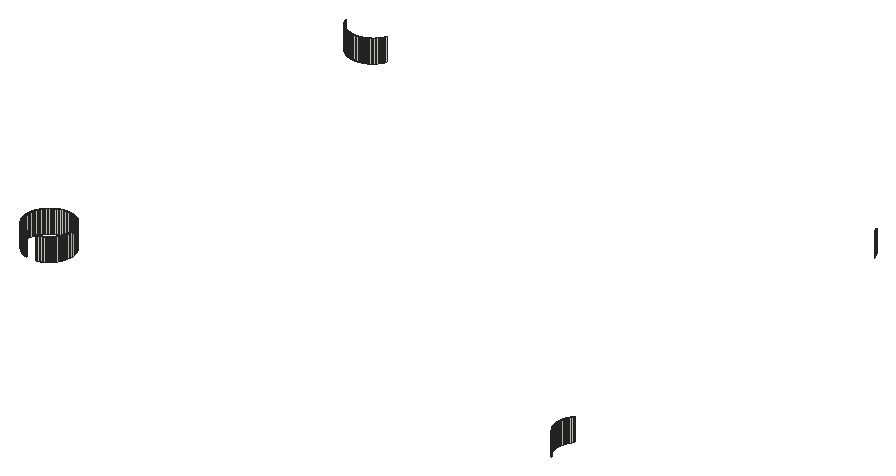
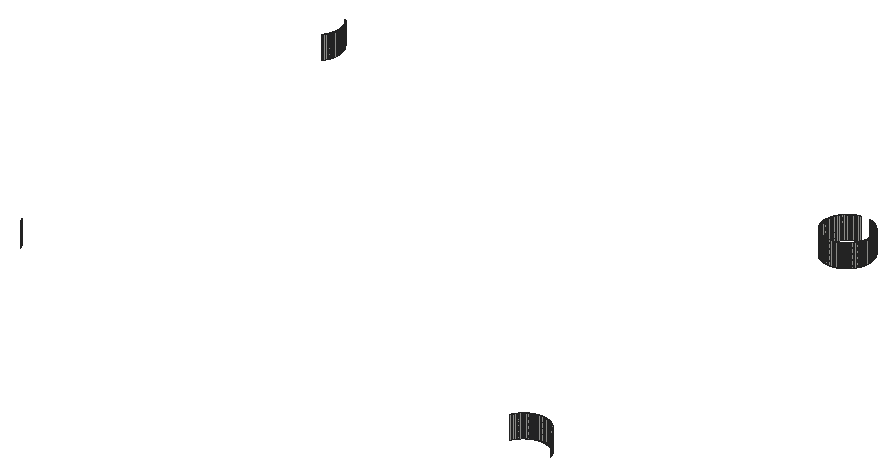
# SketchUp Ruby script. Lengths in inches.
U = 1.inch
M = Sketchup.active_model
def pt(a) = Geom::Point3d.new(a.map { |v| v * U })
def face(e, loops, mat)
  f = e.add_face(loops[0].map { |a| pt(a) })
  loops[1..].each { |l| e.add_face(l.map { |a| pt(a) }).erase! }
  f.material = f.back_material = mat if mat
  f
end
# faces: each face lists its corners as indices into pts; further lists are holes
def faces(e, pts, list, mat = nil) = list.each { |f| face(e, (f[0].is_a?(Array) ? f : [f]).map { |l| l.map { |i| pts[i] } }, mat) }
# xy, xz, yz: faces in a plane at the given z, y or x. An outline is a flat list of corners, or four numbers for a rectangle; further outlines are holes
def ring(l) = l.size == 4 ? [[l[0], l[1]], [l[2], l[1]], [l[2], l[3]], [l[0], l[3]]] : l.each_slice(2).to_a
def flat(e, list, mat, &to3) = list.each { |f| face(e, (f[0].is_a?(Array) ? f : [f]).map { |l| ring(l).map { |u, v| to3.(u, v) } }, mat) }
def xy(e, z, list, mat = nil) = flat(e, list, mat) { |x, y| [x, y, z] }
def xz(e, y, list, mat = nil) = flat(e, list, mat) { |x, z| [x, y, z] }
def yz(e, x, list, mat = nil) = flat(e, list, mat) { |y, z| [x, y, z] }
def lines(e, pts, list) = list.each { |a, b| e.add_line(pt(pts[a]), pt(pts[b])) }
# prism: a flat outline (further loops are holes) pulled along v
def prism(e, loops, v, mat = nil)
  f = face(e, loops, mat); d = Geom::Vector3d.new(v.map { |x| x * U })
  f.pushpull(f.normal.samedirection?(d) ? d.length : -d.length)
end
def box(e, o, s, mat = nil) = prism(e, [[o, [o[0] + s[0], o[1], o[2]], [o[0] + s[0], o[1] + s[1], o[2]], [o[0], o[1] + s[1], o[2]]]], [0, 0, s[2]], mat)
def at(x, y, z, deg = 0) = Geom::Transformation.translation(pt([x, y, z])) * Geom::Transformation.rotation(ORIGIN, Z_AXIS, deg.degrees)
def axes(o, x, y, z) = Geom::Transformation.new([*x, 0, *y, 0, *z, 0, *pt(o).to_a, 1])
def part(name) = M.definitions.add(name)
# library, detail: a bought-in or finely detailed component or shape, given as its bounding box
def library(name, o, s) = part(name).tap { |d| box(d.entities, o, s) }
def detail(e, o, s) = box(e.add_group.entities, o, s)
def put(e, d, t, mat = nil) = e.add_instance(d, t).tap { |i| i.material = mat if mat }
def group(e, t, mat = nil) = e.add_group.tap { |g| g.transformation = t; g.material = mat if mat }.entities
root = M.entities
xz(root,125,[[30.34,129,30.42,132],[30.42,129,30.5,132],[30.5,129,30.58,132],[30.58,129,30.66,132]])
xz(root,172.75,[[30.34,129,30.42,132],[30.42,129,30.5,132],[30.5,129,30.58,132],[30.58,129,30.66,132]])
yz(root,27.5,[[121.84,129,121.92,132],[121.92,129,122,132],[122,129,122.08,132],[122.08,129,122.16,132]])
yz(root,33.5,[[121.84,129,121.92,132],[121.92,129,122,132],[122,129,122.08,132],[122.08,129,122.16,132]])
yz(root,98,[[121.84,129,121.92,132],[121.92,129,122,132],[122,129,122.08,132],[122.08,129,122.16,132]])
p = [[29.57,119.15,129],[29.5,119.17,129],[29.5,119.17,132],[29.57,119.15,132],[29.72,119.1,129],[29.65,119.125,129],
  [29.65,119.125,132],[29.72,119.1,132],[29.8,119.08,129],[29.8,119.08,132],[29.875,119.07,129],[29.875,119.07,132],
  [31.125,119.07,129],[31.05,119.05,129],[31.05,119.05,132],[31.125,119.07,132],[31.2,119.08,129],[31.2,119.08,132],
  [31.28,119.1,129],[31.28,119.1,132],[31.35,119.125,129],[31.35,119.125,132],[31.43,119.15,129],[31.43,119.15,132],
  [31.5,119.17,129],[31.5,119.17,132],[29.35,119.23,129],[29.28,119.26,129],[29.28,119.26,132],[29.35,119.23,132],
  [29.42,119.2,129],[29.42,119.2,132],[31.58,119.2,129],[31.58,119.2,132],[31.65,119.23,129],[31.65,119.23,132],
  [31.72,119.26,129],[31.72,119.26,132],[29.21,119.29,129],[29.14,119.33,129],[29.14,119.33,132],[29.21,119.29,132],
  [29.07,119.36,129],[29.07,119.36,132],[31.79,119.29,129],[31.79,119.29,132],[31.86,119.33,129],[31.86,119.33,132],
  [31.93,119.36,129],[31.93,119.36,132],[29,119.4,129],[28.93,119.44,129],[28.93,119.44,132],[29,119.4,132],
  [28.87,119.48,129],[28.87,119.48,132],[32,119.4,129],[32,119.4,132],[32.07,119.44,129],[32.07,119.44,132],
  [32.13,119.48,129],[32.13,119.48,132],[28.8,119.53,129],[28.74,119.57,129],[28.74,119.57,132],[28.8,119.53,132],
  [32.2,119.53,129],[32.2,119.53,132],[32.26,119.57,129],[32.26,119.57,132],[28.67,119.62,129],[28.61,119.67,129],
  [28.61,119.67,132],[28.67,119.62,132],[32.33,119.62,129],[32.33,119.62,132],[32.39,119.67,129],[32.39,119.67,132],
  [28.55,119.72,129],[28.49,119.77,129],[28.49,119.77,132],[28.55,119.72,132],[32.45,119.72,129],[32.45,119.72,132],
  [32.51,119.77,129],[32.51,119.77,132],[28.43,119.82,129],[28.43,119.82,132],[28.38,119.88,129],[28.38,119.88,132],
  [32.57,119.82,129],[32.57,119.82,132],[32.62,119.88,129],[32.62,119.88,132],[28.32,119.93,129],[28.32,119.93,132],
  [28.27,119.99,129],[28.27,119.99,132],[32.68,119.93,129],[32.68,119.93,132],[32.73,119.99,129],[32.73,119.99,132],
  [28.22,120.05,129],[28.22,120.05,132],[32.78,120.05,129],[32.78,120.05,132],[28.17,120.11,129],[28.12,120.17,129],
  [28.12,120.17,132],[28.17,120.11,132],[32.83,120.11,129],[32.83,120.11,132],[32.88,120.17,129],[32.88,120.17,132],
  [98.67,120.11,129],[98.62,120.17,129],[98.62,120.17,132],[98.67,120.11,132],[98.72,120.05,129],[98.72,120.05,132],
  [28.07,120.24,129],[28.03,120.3,129],[28.03,120.3,132],[28.07,120.24,132],[32.93,120.24,129],[32.93,120.24,132],
  [32.97,120.3,129],[32.97,120.3,132],[98.57,120.24,129],[98.53,120.3,129],[98.53,120.3,132],[98.57,120.24,132],
  [27.98,120.37,129],[27.98,120.37,132],[33.02,120.37,129],[33.02,120.37,132],[98.48,120.37,129],[98.48,120.37,132],
  [27.94,120.43,129],[27.94,120.43,132],[27.9,120.5,129],[27.9,120.5,132],[33.06,120.43,129],[33.06,120.43,132],
  [33.1,120.5,129],[33.1,120.5,132],[98.44,120.43,129],[98.44,120.43,132],[98.4,120.5,129],[98.4,120.5,132],
  [27.86,120.57,129],[27.86,120.57,132],[33.14,120.57,129],[33.14,120.57,132],[98.36,120.57,129],[98.36,120.57,132],
  [27.83,120.64,129],[27.83,120.64,132],[27.79,120.71,129],[27.79,120.71,132],[33.17,120.64,129],[33.17,120.64,132],
  [33.21,120.71,129],[33.21,120.71,132],[98.33,120.64,129],[98.33,120.64,132],[98.29,120.71,129],[98.29,120.71,132],
  [27.76,120.78,129],[27.76,120.78,132],[33.24,120.78,129],[33.24,120.78,132],[98.26,120.78,129],[98.26,120.78,132],
  [27.73,120.85,129],[27.73,120.85,132],[33.27,120.85,129],[33.27,120.85,132],[98.23,120.85,129],[98.23,120.85,132],
  [27.7,120.92,129],[27.7,120.92,132],[27.67,121,129],[27.67,121,132],[33.3,120.92,129],[33.3,120.92,132],
  [33.33,121,129],[33.33,121,132],[98.2,120.92,129],[98.2,120.92,132],[98.17,121,129],[98.17,121,132],
  [27.65,121.07,129],[27.65,121.07,132],[33.35,121.07,129],[33.35,121.07,132],[98.15,121.07,129],[98.15,121.07,132],
  [27.625,121.15,129],[27.625,121.15,132],[27.6,121.22,129],[27.6,121.22,132],[33.375,121.15,129],[33.375,121.15,132],
  [33.4,121.22,129],[33.4,121.22,132],[98.125,121.15,129],[98.125,121.15,132],[98.1,121.22,129],[98.1,121.22,132],
  [27.58,121.3,129],[27.58,121.3,132],[33.42,121.3,129],[33.42,121.3,132],[98.08,121.3,129],[98.08,121.3,132],
  [27.57,121.375,129],[27.57,121.375,132],[33.43,121.375,129],[33.43,121.375,132],[98.07,121.375,129],[98.07,121.375,132],
  [27.55,121.45,129],[27.55,121.45,132],[33.45,121.45,129],[33.45,121.45,132],[98.05,121.45,129],[98.05,121.45,132],
  [27.54,121.53,129],[27.54,121.53,132],[27.53,121.61,129],[27.53,121.61,132],[33.46,121.53,129],[33.46,121.53,132],
  [33.47,121.61,129],[33.47,121.61,132],[98.04,121.53,129],[98.04,121.53,132],[98.03,121.61,129],[98.03,121.61,132],
  [27.52,121.6875,129],[27.52,121.6875,132],[33.48,121.6875,129],[33.48,121.6875,132],[98.02,121.6875,129],[98.02,121.6875,132],
  [27.51,121.76,129],[27.51,121.76,132],[33.49,121.76,129],[33.49,121.76,132],[98.01,121.76,129],[98.01,121.76,132],
  [27.5,121.84,129],[27.5,121.84,132],[33.5,121.84,129],[33.5,121.84,132],[98,121.84,129],[98,121.84,132],
  [27.5,122.16,129],[27.51,122.24,129],[27.51,122.24,132],[27.5,122.16,132],[27.52,122.3125,129],[27.52,122.3125,132],
  [33.49,122.24,129],[33.5,122.16,129],[33.5,122.16,132],[33.49,122.24,132],[33.48,122.3125,129],[33.48,122.3125,132],
  [98,122.16,129],[98.01,122.24,129],[98.01,122.24,132],[98,122.16,132],[98.02,122.3125,129],[98.02,122.3125,132],
  [27.53,122.39,129],[27.53,122.39,132],[33.47,122.39,129],[33.47,122.39,132],[98.03,122.39,129],[98.03,122.39,132],
  [27.54,122.47,129],[27.54,122.47,132],[33.46,122.47,129],[33.46,122.47,132],[98.04,122.47,129],[98.04,122.47,132],
  [27.55,122.55,129],[27.55,122.55,132],[27.57,122.625,129],[27.57,122.625,132],[33.45,122.55,129],[33.45,122.55,132],
  [33.43,122.625,129],[33.43,122.625,132],[98.05,122.55,129],[98.05,122.55,132],[98.07,122.625,129],[98.07,122.625,132],
  [27.58,122.7,129],[27.58,122.7,132],[33.42,122.7,129],[33.42,122.7,132],[98.08,122.7,129],[98.08,122.7,132],
  [27.6,122.78,129],[27.6,122.78,132],[33.4,122.78,129],[33.4,122.78,132],[98.1,122.78,129],[98.1,122.78,132],
  [27.625,122.85,129],[27.625,122.85,132],[33.375,122.85,129],[33.375,122.85,132],[98.125,122.85,129],[98.125,122.85,132],
  [27.65,122.93,129],[27.65,122.93,132],[27.67,123,129],[27.67,123,132],[33.33,123,129],[33.35,122.93,129],
  [33.35,122.93,132],[33.33,123,132],[98.15,122.93,129],[98.15,122.93,132],[98.17,123,129],[98.17,123,132],
  [27.7,123.08,129],[27.7,123.08,132],[33.3,123.08,129],[33.3,123.08,132],[98.2,123.08,129],[98.2,123.08,132],
  [27.73,123.15,129],[27.73,123.15,132],[27.76,123.22,129],[27.76,123.22,132],[33.24,123.22,129],[33.27,123.15,129],
  [33.27,123.15,132],[33.24,123.22,132],[98.23,123.15,129],[98.23,123.15,132],[98.26,123.22,129],[98.26,123.22,132],
  [27.79,123.29,129],[27.79,123.29,132],[33.21,123.29,129],[33.21,123.29,132],[98.29,123.29,129],[98.29,123.29,132],
  [27.83,123.36,129],[27.83,123.36,132],[33.17,123.36,129],[33.17,123.36,132],[98.33,123.36,129],[98.33,123.36,132],
  [27.86,123.43,129],[27.86,123.43,132],[27.9,123.5,129],[27.9,123.5,132],[33.14,123.43,129],[33.14,123.43,132],
  [33.1,123.5,129],[33.1,123.5,132],[98.36,123.43,129],[98.36,123.43,132],[98.4,123.5,129],[98.4,123.5,132],
  [27.94,123.57,129],[27.94,123.57,132],[33.06,123.57,129],[33.06,123.57,132],[98.44,123.57,129],[98.44,123.57,132],
  [27.98,123.63,129],[27.98,123.63,132],[28.03,123.7,129],[28.03,123.7,132],[33.02,123.63,129],[33.02,123.63,132],
  [32.97,123.7,129],[32.97,123.7,132],[98.48,123.63,129],[98.48,123.63,132],[98.53,123.7,129],[98.53,123.7,132],
  [28.07,123.76,129],[28.07,123.76,132],[32.93,123.76,129],[32.93,123.76,132],[98.57,123.76,129],[98.57,123.76,132],
  [28.12,123.83,129],[28.12,123.83,132],[28.17,123.89,129],[28.17,123.89,132],[32.83,123.89,129],[32.88,123.83,129],
  [32.88,123.83,132],[32.83,123.89,132],[98.62,123.83,129],[98.62,123.83,132],[98.67,123.89,129],[98.67,123.89,132],
  [28.22,123.95,129],[28.22,123.95,132],[28.27,124.01,129],[28.27,124.01,132],[32.73,124.01,129],[32.78,123.95,129],
  [32.78,123.95,132],[32.73,124.01,132],[98.72,123.95,129],[98.72,123.95,132],[28.32,124.07,129],[28.32,124.07,132],
  [32.68,124.07,129],[32.68,124.07,132],[28.38,124.12,129],[28.38,124.12,132],[28.43,124.18,129],[28.43,124.18,132],
  [32.62,124.12,129],[32.62,124.12,132],[32.57,124.18,129],[32.57,124.18,132],[28.49,124.23,129],[28.49,124.23,132],
  [28.55,124.28,129],[28.55,124.28,132],[32.45,124.28,129],[32.51,124.23,129],[32.51,124.23,132],[32.45,124.28,132],
  [28.61,124.33,129],[28.61,124.33,132],[28.67,124.38,129],[28.67,124.38,132],[32.33,124.38,129],[32.39,124.33,129],
  [32.39,124.33,132],[32.33,124.38,132],[28.74,124.43,129],[28.74,124.43,132],[28.8,124.47,129],[28.8,124.47,132],
  [32.2,124.47,129],[32.26,124.43,129],[32.26,124.43,132],[32.2,124.47,132],[28.87,124.52,129],[28.87,124.52,132],
  [28.93,124.56,129],[28.93,124.56,132],[32.13,124.52,129],[32.13,124.52,132],[32.07,124.56,129],[32.07,124.56,132],
  [29,124.6,129],[29,124.6,132],[29.07,124.64,129],[29.07,124.64,132],[29.14,124.67,129],[29.14,124.67,132],
  [31.93,124.64,129],[32,124.6,129],[32,124.6,132],[31.93,124.64,132],[31.86,124.67,129],[31.86,124.67,132],
  [29.21,124.71,129],[29.21,124.71,132],[29.28,124.74,129],[29.28,124.74,132],[29.35,124.77,129],[29.35,124.77,132],
  [31.65,124.77,129],[31.72,124.74,129],[31.72,124.74,132],[31.65,124.77,132],[31.79,124.71,129],[31.79,124.71,132],
  [29.42,124.8,129],[29.42,124.8,132],[29.5,124.83,129],[29.5,124.83,132],[29.57,124.85,129],[29.57,124.85,132],
  [31.43,124.85,129],[31.5,124.83,129],[31.5,124.83,132],[31.43,124.85,132],[31.58,124.8,129],[31.58,124.8,132],
  [29.65,124.875,129],[29.65,124.875,132],[29.72,124.9,129],[29.72,124.9,132],[29.8,124.92,129],[29.8,124.92,132],
  [29.875,124.93,129],[29.875,124.93,132],[29.95,124.95,129],[29.95,124.95,132],[30.03,124.96,129],[30.03,124.96,132],
  [31.05,124.95,129],[31.125,124.93,129],[31.125,124.93,132],[31.05,124.95,132],[30.97,124.96,129],[30.97,124.96,132],
  [31.2,124.92,129],[31.2,124.92,132],[31.28,124.9,129],[31.28,124.9,132],[31.35,124.875,129],[31.35,124.875,132],
  [30.11,124.97,129],[30.11,124.97,132],[30.1875,124.98,129],[30.1875,124.98,132],[30.26,124.99,129],[30.26,124.99,132],
  [30.34,125,129],[30.34,125,132],[30.74,124.99,129],[30.8125,124.98,129],[30.8125,124.98,132],[30.74,124.99,132],
  [30.66,125,129],[30.66,125,132],[30.89,124.97,129],[30.89,124.97,132],[29.8,172.83,129],[29.72,172.85,129],
  [29.72,172.85,132],[29.8,172.83,132],[29.875,172.82,129],[29.875,172.82,132],[29.95,172.8,129],[29.95,172.8,132],
  [30.11,172.78,129],[30.03,172.79,129],[30.03,172.79,132],[30.11,172.78,132],[30.1875,172.77,129],[30.1875,172.77,132],
  [30.26,172.76,129],[30.26,172.76,132],[30.34,172.75,129],[30.34,172.75,132],[30.74,172.76,129],[30.66,172.75,129],
  [30.66,172.75,132],[30.74,172.76,132],[30.8125,172.77,129],[30.8125,172.77,132],[30.89,172.78,129],[30.89,172.78,132],
  [30.97,172.79,129],[30.97,172.79,132],[31.05,172.8,129],[31.05,172.8,132],[31.125,172.82,129],[31.125,172.82,132],
  [31.2,172.83,129],[31.2,172.83,132],[31.28,172.85,129],[31.28,172.85,132],[29.5,172.92,129],[29.42,172.95,129],
  [29.42,172.95,132],[29.5,172.92,132],[29.35,172.98,129],[29.35,172.98,132],[29.57,172.9,129],[29.57,172.9,132],
  [29.65,172.875,129],[29.65,172.875,132],[31.35,172.875,129],[31.35,172.875,132],[31.43,172.9,129],[31.43,172.9,132],
  [31.5,172.92,129],[31.5,172.92,132],[31.58,172.95,129],[31.58,172.95,132],[31.65,172.98,129],[31.65,172.98,132],
  [29.21,173.04,129],[29.14,173.08,129],[29.14,173.08,132],[29.21,173.04,132],[29.28,173.01,129],[29.28,173.01,132],
  [31.72,173.01,129],[31.72,173.01,132],[31.79,173.04,129],[31.79,173.04,132],[31.86,173.08,129],[31.86,173.08,132],
  [29.07,173.11,129],[29,173.15,129],[29,173.15,132],[29.07,173.11,132],[31.93,173.11,129],[31.93,173.11,132],
  [32,173.15,129],[32,173.15,132],[28.87,173.23,129],[28.8,173.28,129],[28.8,173.28,132],[28.87,173.23,132],
  [28.93,173.19,129],[28.93,173.19,132],[32.07,173.19,129],[32.07,173.19,132],[32.13,173.23,129],[32.13,173.23,132],
  [32.2,173.28,129],[32.2,173.28,132],[28.74,173.32,129],[28.74,173.32,132],[28.67,173.37,129],[28.67,173.37,132],
  [32.26,173.32,129],[32.26,173.32,132],[32.33,173.37,129],[32.33,173.37,132],[28.61,173.42,129],[28.61,173.42,132],
  [28.55,173.47,129],[28.55,173.47,132],[32.39,173.42,129],[32.39,173.42,132],[32.45,173.47,129],[32.45,173.47,132],
  [28.49,173.52,129],[28.43,173.57,129],[28.43,173.57,132],[28.49,173.52,132],[32.51,173.52,129],[32.51,173.52,132],
  [32.57,173.57,129],[32.57,173.57,132],[28.38,173.63,129],[28.32,173.68,129],[28.32,173.68,132],[28.38,173.63,132],
  [32.62,173.63,129],[32.62,173.63,132],[32.68,173.68,129],[32.68,173.68,132],[28.27,173.74,129],[28.22,173.8,129],
  [28.22,173.8,132],[28.27,173.74,132],[32.73,173.74,129],[32.73,173.74,132],[32.78,173.8,129],[32.78,173.8,132],
  [28.17,173.86,129],[28.17,173.86,132],[32.83,173.86,129],[32.83,173.86,132],[28.12,173.92,129],[28.12,173.92,132],
  [28.07,173.99,129],[28.07,173.99,132],[32.88,173.92,129],[32.88,173.92,132],[32.93,173.99,129],[32.93,173.99,132],
  [98.67,173.86,129],[98.62,173.92,129],[98.62,173.92,132],[98.67,173.86,132],[98.57,173.99,129],[98.57,173.99,132],
  [28.03,174.05,129],[28.03,174.05,132],[32.97,174.05,129],[32.97,174.05,132],[98.53,174.05,129],[98.53,174.05,132],
  [27.98,174.12,129],[27.94,174.18,129],[27.94,174.18,132],[27.98,174.12,132],[33.02,174.12,129],[33.02,174.12,132],
  [33.06,174.18,129],[33.06,174.18,132],[98.48,174.12,129],[98.44,174.18,129],[98.44,174.18,132],[98.48,174.12,132],
  [27.9,174.25,129],[27.9,174.25,132],[27.86,174.32,129],[27.86,174.32,132],[33.1,174.25,129],[33.1,174.25,132],
  [98.4,174.25,129],[98.4,174.25,132],[98.36,174.32,129],[98.36,174.32,132],[27.83,174.39,129],[27.83,174.39,132],
  [33.14,174.32,129],[33.14,174.32,132],[33.17,174.39,129],[33.17,174.39,132],[98.33,174.39,129],[98.33,174.39,132],
  [27.79,174.46,129],[27.79,174.46,132],[33.21,174.46,129],[33.21,174.46,132],[98.29,174.46,129],[98.29,174.46,132],
  [27.76,174.53,129],[27.73,174.6,129],[27.73,174.6,132],[27.76,174.53,132],[33.24,174.53,129],[33.24,174.53,132],
  [98.26,174.53,129],[98.23,174.6,129],[98.23,174.6,132],[98.26,174.53,132]]
faces(root,p,[[0,1,2,3],[4,5,6,7],[5,0,3,6],[8,4,7,9],[10,8,9,11],[12,13,14,15],[16,12,15,17],[18,16,17,19],
  [20,18,19,21],[22,20,21,23],[24,22,23,25],[26,27,28,29],[1,30,31,2],[30,26,29,31],[32,24,25,33],[34,32,33,35],
  [36,34,35,37],[38,39,40,41],[39,42,43,40],[27,38,41,28],[44,36,37,45],[46,44,45,47],[48,46,47,49],[50,51,52,53],
  [51,54,55,52],[42,50,53,43],[56,48,49,57],[58,56,57,59],[60,58,59,61],[62,63,64,65],[54,62,65,55],[66,60,61,67],
  [68,66,67,69],[70,71,72,73],[63,70,73,64],[74,68,69,75],[76,74,75,77],[78,79,80,81],[71,78,81,72],[82,76,77,83],
  [84,82,83,85],[79,86,87,80],[86,88,89,87],[90,84,85,91],[92,90,91,93],[88,94,95,89],[94,96,97,95],[98,92,93,99],
  [100,98,99,101],[96,102,103,97],[104,100,101,105],[106,107,108,109],[102,106,109,103],[110,104,105,111],[112,110,111,113],[114,115,116,117],
  [118,114,117,119],[120,121,122,123],[107,120,123,108],[124,112,113,125],[126,124,125,127],[128,129,130,131],[115,128,131,116],[121,132,133,122],
  [134,126,127,135],[129,136,137,130],[132,138,139,133],[138,140,141,139],[142,134,135,143],[144,142,143,145],[136,146,147,137],[146,148,149,147],
  [140,150,151,141],[152,144,145,153],[148,154,155,149],[150,156,157,151],[156,158,159,157],[160,152,153,161],[162,160,161,163],[154,164,165,155],
  [164,166,167,165],[158,168,169,159],[170,162,163,171],[166,172,173,167],[168,174,175,169],[176,170,171,177],[172,178,179,173],[174,180,181,175],
  [180,182,183,181],[184,176,177,185],[186,184,185,187],[178,188,189,179],[188,190,191,189],[182,192,193,183],[194,186,187,195],[190,196,197,191],
  [192,198,199,193],[198,200,201,199],[202,194,195,203],[204,202,203,205],[196,206,207,197],[206,208,209,207],[200,210,211,201],[212,204,205,213],
  [208,214,215,209],[210,216,217,211],[218,212,213,219],[214,220,221,215],[216,222,223,217],[224,218,219,225],[220,226,227,221],[222,228,229,223],
  [228,230,231,229],[232,224,225,233],[234,232,233,235],[226,236,237,227],[236,238,239,237],[230,240,241,231],[242,234,235,243],[238,244,245,239],
  [240,246,247,241],[248,242,243,249],[244,250,251,245],[246,252,253,247],[254,248,249,255],[250,256,257,251],[258,259,260,261],[259,262,263,260],
  [264,265,266,267],[268,264,267,269],[270,271,272,273],[271,274,275,272],[262,276,277,263],[278,268,269,279],[274,280,281,275],[276,282,283,277],
  [284,278,279,285],[280,286,287,281],[282,288,289,283],[288,290,291,289],[292,284,285,293],[294,292,293,295],[286,296,297,287],[296,298,299,297],
  [290,300,301,291],[302,294,295,303],[298,304,305,299],[300,306,307,301],[308,302,303,309],[304,310,311,305],[306,312,313,307],[314,308,309,315],
  [310,316,317,311],[312,318,319,313],[318,320,321,319],[322,323,324,325],[323,314,315,324],[316,326,327,317],[326,328,329,327],[320,330,331,321],
  [332,322,325,333],[328,334,335,329],[330,336,337,331],[336,338,339,337],[340,341,342,343],[341,332,333,342],[334,344,345,335],[344,346,347,345],
  [338,348,349,339],[350,340,343,351],[346,352,353,347],[348,354,355,349],[356,350,351,357],[352,358,359,353],[354,360,361,355],[360,362,363,361],
  [364,356,357,365],[366,364,365,367],[358,368,369,359],[368,370,371,369],[362,372,373,363],[374,366,367,375],[370,376,377,371],[372,378,379,373],
  [378,380,381,379],[382,374,375,383],[384,382,383,385],[376,386,387,377],[386,388,389,387],[380,390,391,381],[392,384,385,393],[388,394,395,389],
  [390,396,397,391],[396,398,399,397],[400,401,402,403],[401,392,393,402],[394,404,405,395],[404,406,407,405],[398,408,409,399],[408,410,411,409],
  [412,413,414,415],[413,400,403,414],[406,416,417,407],[410,418,419,411],[420,412,415,421],[418,422,423,419],[422,424,425,423],[426,420,421,427],
  [428,426,427,429],[424,430,431,425],[430,432,433,431],[434,435,436,437],[435,428,429,436],[432,438,439,433],[438,440,441,439],[442,443,444,445],
  [443,434,437,444],[440,446,447,441],[446,448,449,447],[450,451,452,453],[451,442,445,452],[448,454,455,449],[454,456,457,455],[458,450,453,459],
  [460,458,459,461],[456,462,463,457],[462,464,465,463],[464,466,467,465],[468,469,470,471],[472,468,471,473],[469,460,461,470],[466,474,475,467],
  [474,476,477,475],[476,478,479,477],[480,481,482,483],[481,484,485,482],[484,472,473,485],[478,486,487,479],[486,488,489,487],[488,490,491,489],
  [492,493,494,495],[493,496,497,494],[496,480,483,497],[490,498,499,491],[498,500,501,499],[500,502,503,501],[502,504,505,503],[504,506,507,505],
  [506,508,509,507],[510,511,512,513],[514,510,513,515],[511,516,517,512],[516,518,519,517],[518,520,521,519],[520,492,495,521],[508,522,523,509],
  [522,524,525,523],[524,526,527,525],[526,528,529,527],[530,531,532,533],[534,530,533,535],[531,536,537,532],[536,514,515,537],[538,539,540,541],
  [542,538,541,543],[544,542,543,545],[546,547,548,549],[547,544,545,548],[550,546,549,551],[552,550,551,553],[554,552,553,555],[556,557,558,559],
  [560,556,559,561],[562,560,561,563],[564,562,563,565],[566,564,565,567],[568,566,567,569],[570,568,569,571],[572,570,571,573],[574,575,576,577],
  [575,578,579,576],[580,574,577,581],[539,582,583,540],[582,580,581,583],[584,572,573,585],[586,584,585,587],[588,586,587,589],[590,588,589,591],
  [592,590,591,593],[594,595,596,597],[598,594,597,599],[578,598,599,579],[600,592,593,601],[602,600,601,603],[604,602,603,605],[606,607,608,609],
  [595,606,609,596],[610,604,605,611],[612,610,611,613],[614,615,616,617],[607,618,619,608],[618,614,617,619],[620,612,613,621],[622,620,621,623],
  [624,622,623,625],[615,626,627,616],[626,628,629,627],[630,624,625,631],[632,630,631,633],[628,634,635,629],[634,636,637,635],[638,632,633,639],
  [640,638,639,641],[642,643,644,645],[636,642,645,637],[646,640,641,647],[648,646,647,649],[650,651,652,653],[643,650,653,644],[654,648,649,655],
  [656,654,655,657],[658,659,660,661],[651,658,661,652],[662,656,657,663],[664,662,663,665],[659,666,667,660],[668,664,665,669],[666,670,671,667],
  [670,672,673,671],[674,668,669,675],[676,674,675,677],[678,679,680,681],[679,682,683,680],[672,684,685,673],[686,676,677,687],[682,688,689,683],
  [690,691,692,693],[684,690,693,685],[694,686,687,695],[696,694,695,697],[698,699,700,701],[688,698,701,689],[691,702,703,692],[702,704,705,703],
  [706,696,697,707],[699,708,709,700],[708,710,711,709],[704,712,713,705],[714,706,707,715],[716,714,715,717],[710,718,719,711],[712,720,721,713],
  [722,716,717,723],[718,724,725,719],[726,727,728,729],[720,726,729,721],[730,722,723,731],[732,733,734,735],[724,732,735,725]])
